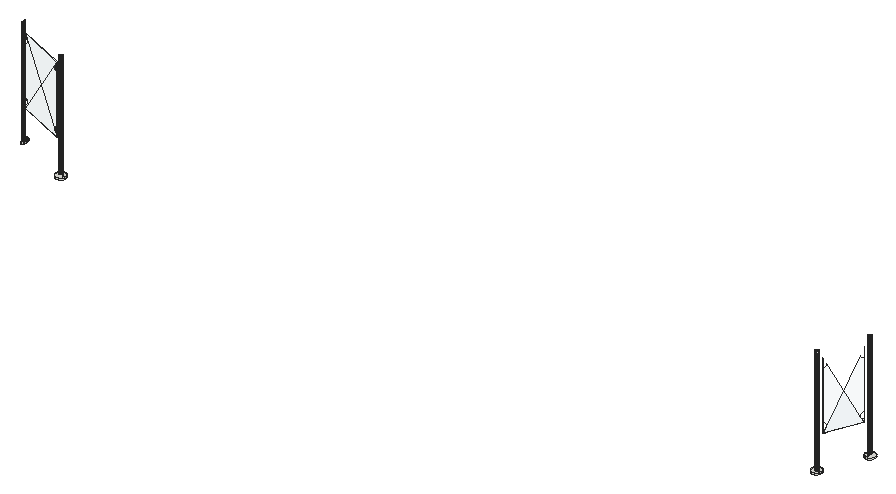
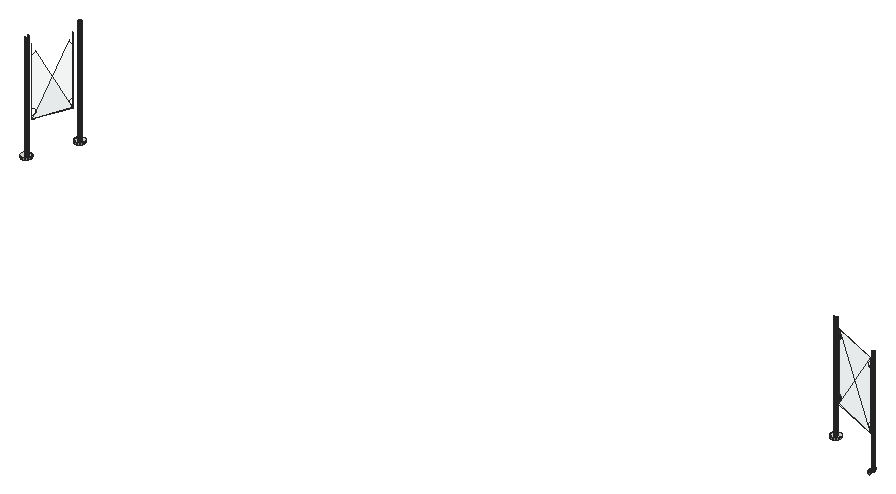
# SketchUp Ruby script. Lengths in inches.
U = 1.inch
M = Sketchup.active_model
def pt(a) = Geom::Point3d.new(a.map { |v| v * U })
def face(e, loops, mat)
  f = e.add_face(loops[0].map { |a| pt(a) })
  loops[1..].each { |l| e.add_face(l.map { |a| pt(a) }).erase! }
  f.material = f.back_material = mat if mat
  f
end
# faces: each face lists its corners as indices into pts; further lists are holes
def faces(e, pts, list, mat = nil) = list.each { |f| face(e, (f[0].is_a?(Array) ? f : [f]).map { |l| l.map { |i| pts[i] } }, mat) }
# xy, xz, yz: faces in a plane at the given z, y or x. An outline is a flat list of corners, or four numbers for a rectangle; further outlines are holes
def ring(l) = l.size == 4 ? [[l[0], l[1]], [l[2], l[1]], [l[2], l[3]], [l[0], l[3]]] : l.each_slice(2).to_a
def flat(e, list, mat, &to3) = list.each { |f| face(e, (f[0].is_a?(Array) ? f : [f]).map { |l| ring(l).map { |u, v| to3.(u, v) } }, mat) }
def xy(e, z, list, mat = nil) = flat(e, list, mat) { |x, y| [x, y, z] }
def xz(e, y, list, mat = nil) = flat(e, list, mat) { |x, z| [x, y, z] }
def yz(e, x, list, mat = nil) = flat(e, list, mat) { |y, z| [x, y, z] }
def lines(e, pts, list) = list.each { |a, b| e.add_line(pt(pts[a]), pt(pts[b])) }
# prism: a flat outline (further loops are holes) pulled along v
def prism(e, loops, v, mat = nil)
  f = face(e, loops, mat); d = Geom::Vector3d.new(v.map { |x| x * U })
  f.pushpull(f.normal.samedirection?(d) ? d.length : -d.length)
end
def box(e, o, s, mat = nil) = prism(e, [[o, [o[0] + s[0], o[1], o[2]], [o[0] + s[0], o[1] + s[1], o[2]], [o[0], o[1] + s[1], o[2]]]], [0, 0, s[2]], mat)
def at(x, y, z, deg = 0) = Geom::Transformation.translation(pt([x, y, z])) * Geom::Transformation.rotation(ORIGIN, Z_AXIS, deg.degrees)
def axes(o, x, y, z) = Geom::Transformation.new([*x, 0, *y, 0, *z, 0, *pt(o).to_a, 1])
def part(name) = M.definitions.add(name)
# library, detail: a bought-in or finely detailed component or shape, given as its bounding box
def library(name, o, s) = part(name).tap { |d| box(d.entities, o, s) }
def detail(e, o, s) = box(e.add_group.entities, o, s)
def put(e, d, t, mat = nil) = e.add_instance(d, t).tap { |i| i.material = mat if mat }
def group(e, t, mat = nil) = e.add_group.tap { |g| g.transformation = t; g.material = mat if mat }.entities
root = M.entities
M.materials.add("Glass_Safety_01").color = [204, 235, 244]
M.materials["Glass_Safety_01"].alpha = 0.1
M.materials.add("[Color_000]").color = [255, 255, 255]
xy(root,321.27,[[[632.17,624.43,632.57,624.51,632.94,624.69,633.25,624.97,633.47,625.31,633.6,625.7,633.63,626.11,633.55,626.51,633.36,626.88,633.09,627.1875,632.74,627.41,632.35,627.54,631.94,627.57,631.54,627.49,631.17,627.3,630.87,627.03,630.64,626.6875,630.62,626.625,630.51,626.3,630.49,625.89,630.57,625.48,630.75,625.11,631.03,624.81,631.37,624.58,631.76,624.45],[632.1,625.37,631.9375,625.38,631.78,625.43,631.64,625.52,631.54,625.64,631.46,625.79,631.43,625.95,631.4375,626.12,631.48,626.25,631.49,626.27,631.58,626.41,631.7,626.52,631.85,626.59,632.01,626.625,632.18,626.62,632.33,626.5625,632.47,626.47,632.58,626.35,632.65,626.2,632.69,626.04,632.68,625.88,632.63,625.75,632.625,625.72,632.53,625.59,632.41,625.48,632.26,625.4]],[[883.4375,625.03,883.84,625.11,884.21,625.3,884.51,625.57,884.74,625.91,884.87,626.3,884.9,626.71,884.8125,627.12,884.63,627.48,884.36,627.79,884.01,628.02,883.62,628.15,883.4,628.16,883.21,628.17,882.81,628.09,882.44,627.91,882.13,627.63,881.91,627.29,881.78,626.9,881.75,626.49,881.84,626.09,882.02,625.72,882.23,625.48,882.29,625.41,882.64,625.18,883.03,625.05],[883.37,625.97,883.21,625.98,883.05,626.03,882.91,626.125,882.8,626.25,882.73,626.39,882.7,626.54,882.7,626.56,882.71,626.72,882.76,626.875,882.85,627.01,882.9375,627.09,882.97,627.12,883.12,627.2,883.28,627.23,883.44,627.22,883.6,627.17,883.74,627.08,883.85,626.95,883.92,626.81,883.95,626.65,883.94,626.48,883.89,626.33,883.8,626.1875,883.68,626.08,883.53,626.01]],[633.49,625.37,633.6,625.7,633.63,626.11,633.55,626.51,633.36,626.88,633.09,627.1875,632.74,627.41,632.35,627.54,631.94,627.57,631.54,627.49,631.17,627.3,630.87,627.03,630.64,626.6875,630.62,626.625,631.48,626.25,631.49,626.27,631.58,626.41,631.7,626.52,631.85,626.59,632.01,626.625,632.18,626.62,632.33,626.5625,632.47,626.47,632.58,626.35,632.65,626.2,632.69,626.04,632.68,625.88,632.63,625.75],[882.23,625.48,882.7,626.54,882.7,626.56,882.71,626.72,882.76,626.875,882.85,627.01,882.9375,627.09,883.4,628.16,883.21,628.17,882.81,628.09,882.44,627.91,882.13,627.63,881.91,627.29,881.78,626.9,881.75,626.49,881.84,626.09,882.02,625.72],[632.63,625.75,632.68,625.88,632.69,626.04,632.65,626.2,632.58,626.35,632.47,626.47,632.33,626.5625,632.18,626.62,632.01,626.625,631.85,626.59,631.7,626.52,631.58,626.41,631.49,626.27,631.48,626.25],
  [882.7,626.54,882.9375,627.09,882.85,627.01,882.76,626.875,882.71,626.72,882.7,626.56],[[889.33,639.9375,889.73,640.02,890.1,640.2,890.41,640.48,890.63,640.82,890.76,641.21,890.79,641.62,890.7,642.02,890.52,642.39,890.25,642.7,889.9,642.92,889.51,643.05,889.1,643.08,888.7,643,888.33,642.8125,888.03,642.54,887.8,642.2,887.67,641.81,887.64,641.4,887.73,640.99,887.91,640.625,888.18,640.32,888.53,640.09,888.92,639.96],[889.26,640.88,889.1,640.89,888.97,640.93,888.94,640.94,888.8,641.03,888.69,641.15,888.62,641.3,888.59,641.46,888.6,641.625,888.65,641.78,888.74,641.92,888.86,642.03,889.01,642.1,889.17,642.14,889.33,642.125,889.47,642.08,889.49,642.07,889.63,641.98,889.74,641.86,889.8125,641.71,889.84,641.55,889.83,641.39,889.78,641.23,889.69,641.1,889.57,640.99,889.42,640.91]],[888.59,640.07,888.97,640.93,888.94,640.94,888.8,641.03,888.69,641.15,888.62,641.3,888.59,641.46,888.6,641.625,888.65,641.78,888.74,641.92,888.86,642.03,889.01,642.1,889.17,642.14,889.33,642.125,889.47,642.08,889.84,642.94,889.51,643.05,889.1,643.08,888.7,643,888.33,642.8125,888.03,642.54,887.8,642.2,887.67,641.81,887.64,641.4,887.73,640.99,887.91,640.625,888.18,640.32,888.53,640.09],[888.97,640.93,889.47,642.08,889.33,642.125,889.17,642.14,889.01,642.1,888.86,642.03,888.74,641.92,888.65,641.78,888.6,641.625,888.59,641.46,888.62,641.3,888.69,641.15,888.8,641.03,888.94,640.94]])
xy(root,321.27,[[883.37,625.97,883.53,626.01,883.68,626.08,883.8,626.1875,883.89,626.33,883.94,626.48,883.95,626.65,883.92,626.81,883.85,626.95,883.74,627.08,883.6,627.17,883.44,627.22,883.28,627.23,883.12,627.2,882.97,627.12,882.9375,627.09,882.85,627.01,882.76,626.875,882.71,626.72,882.7,626.56,882.7,626.54,882.73,626.39,882.8,626.25,882.91,626.125,883.05,626.03,883.21,625.98]],"[Color_000]")
xy(root,321.86,[[632.17,624.43,632.57,624.51,632.94,624.69,633.25,624.97,633.47,625.31,633.6,625.7,633.63,626.11,633.55,626.51,633.36,626.88,633.09,627.1875,632.74,627.41,632.35,627.54,631.94,627.57,631.54,627.49,631.17,627.3,630.87,627.03,630.64,626.6875,630.51,626.3,630.49,625.89,630.57,625.48,630.75,625.11,631.03,624.81,631.37,624.58,631.76,624.45],[883.4375,625.03,883.84,625.11,884.21,625.3,884.51,625.57,884.74,625.91,884.87,626.3,884.9,626.71,884.8125,627.12,884.63,627.48,884.36,627.79,884.01,628.02,883.62,628.15,883.21,628.17,882.81,628.09,882.44,627.91,882.13,627.63,881.91,627.29,881.78,626.9,881.75,626.49,881.84,626.09,882.02,625.72,882.29,625.41,882.64,625.18,883.03,625.05],[889.33,639.9375,889.73,640.02,890.1,640.2,890.41,640.48,890.63,640.82,890.76,641.21,890.79,641.62,890.7,642.02,890.52,642.39,890.25,642.7,889.9,642.92,889.51,643.05,889.1,643.08,888.7,643,888.33,642.8125,888.03,642.54,887.8,642.2,887.67,641.81,887.64,641.4,887.73,640.99,887.91,640.625,888.18,640.32,888.53,640.09,888.92,639.96]])
xy(root,331.9,[[630.38,626.62,614.1875,633.67,614.27,633.85],[630.38,626.62,614.27,633.85,630.46,626.8],[884.14,628.4,883.96,628.47,888.67,639.87],[883.96,628.47,888.49,639.9375,888.67,639.87]],"Glass_Safety_01")
p = [[633.6,625.7,321.27],[633.63,626.11,321.27],[633.63,626.11,321.86],[633.6,625.7,321.86],[630.51,626.3,321.27],[630.49,625.89,321.27],
  [630.49,625.89,321.86],[630.51,626.3,321.86],[632.68,625.88,321.27],[632.69,626.04,321.27],[632.69,626.04,357.27],[632.68,625.88,357.27],
  [884.74,625.91,321.27],[884.87,626.3,321.27],[884.87,626.3,321.86],[884.74,625.91,321.86],[631.4375,626.12,321.27],[631.43,625.95,321.27],
  [631.43,625.95,357.27],[631.4375,626.12,357.27],[632.65,626.2,321.27],[632.65,626.2,357.27],[882.91,626.125,321.27],[883.05,626.03,321.27],
  [883.05,626.03,357.27],[882.91,626.125,357.27],[883.21,625.98,321.27],[883.21,625.98,357.27],[883.37,625.97,321.27],[883.37,625.97,357.27],
  [883.53,626.01,321.27],[883.53,626.01,357.27],[883.68,626.08,321.27],[883.68,626.08,357.27],[631.49,626.27,321.27],[631.48,626.25,321.27],
  [631.49,626.27,357.27],[633.55,626.51,321.27],[633.55,626.51,321.86],[881.75,626.49,321.27],[881.84,626.09,321.27],[881.84,626.09,321.86],
  [881.75,626.49,321.86],[882.8,626.25,321.27],[882.8,626.25,357.27],[883.8,626.1875,321.27],[883.8,626.1875,357.27],[632.58,626.35,321.27],
  [632.58,626.35,357.27],[882.73,626.39,321.27],[882.73,626.39,357.27],[883.89,626.33,321.27],[883.89,626.33,357.27],[630.64,626.6875,321.27],
  [630.62,626.625,321.27],[630.64,626.6875,321.86],[631.58,626.41,321.27],[631.58,626.41,357.27],[883.94,626.48,321.27],[883.94,626.48,357.27],
  [884.9,626.71,321.27],[884.9,626.71,321.86],[631.7,626.52,321.27],[631.7,626.52,357.27],[632.47,626.47,321.27],[632.47,626.47,357.27],
  [882.7,626.56,321.27],[882.7,626.54,321.27],[882.7,626.56,357.27],[631.85,626.59,321.27],[631.85,626.59,357.27],[632.33,626.5625,321.27],
  [632.33,626.5625,357.27],[633.36,626.88,321.27],[633.36,626.88,321.86],[881.78,626.9,321.27],[881.78,626.9,321.86],[883.95,626.65,321.27],
  [883.95,626.65,357.27],[632.01,626.625,321.27],[632.01,626.625,357.27],[632.18,626.62,321.27],[632.18,626.62,357.27],[882.71,626.72,321.27],
  [882.71,626.72,357.27],[883.92,626.81,321.27],[883.92,626.81,357.27],[630.87,627.03,321.27],[630.87,627.03,321.86],[882.76,626.875,321.27],
  [882.76,626.875,357.27],[884.8125,627.12,321.27],[884.8125,627.12,321.86],[883.85,626.95,321.27],[883.85,626.95,357.27],[633.09,627.1875,321.27],
  [633.09,627.1875,321.86],[881.91,627.29,321.27],[881.91,627.29,321.86],[882.85,627.01,321.27],[882.85,627.01,357.27],[631.17,627.3,321.27],
  [631.17,627.3,321.86],[882.97,627.12,321.27],[882.9375,627.09,321.27],[882.97,627.12,357.27],[883.74,627.08,321.27],[883.74,627.08,357.27],
  [883.12,627.2,321.27],[883.12,627.2,357.27],[883.6,627.17,321.27],[883.6,627.17,357.27],[884.63,627.48,321.27],[884.63,627.48,321.86],
  [632.74,627.41,321.27],[632.74,627.41,321.86],[883.28,627.23,321.27],[883.28,627.23,357.27],[883.44,627.22,321.27],[883.44,627.22,357.27],
  [631.54,627.49,321.27],[631.54,627.49,321.86],[882.13,627.63,321.27],[882.13,627.63,321.86],[632.35,627.54,321.27],[632.35,627.54,321.86],
  [631.94,627.57,321.27],[631.94,627.57,321.86],[884.36,627.79,321.27],[884.36,627.79,321.86],[882.44,627.91,321.27],[882.44,627.91,321.86],
  [884.01,628.02,321.27],[884.01,628.02,321.86],[882.81,628.09,321.27],[882.81,628.09,321.86],[883.62,628.15,321.27],[883.62,628.15,321.86],
  [883.21,628.17,321.27],[883.21,628.17,321.86],[883.4,628.16,321.27],[612.9375,633.0625,321.27],[613.3,633.25,321.27],[613.3,633.25,321.86],
  [612.9375,633.0625,321.86],[613.61,633.52,321.27],[613.61,633.52,321.86],[613.84,633.86,321.27],[613.84,633.86,321.86],[613.86,633.92,321.27],
  [613.97,634.25,321.27],[613.97,634.25,321.86],[612.77,634.03,321.27],[612.9,634.14,321.27],[612.9,634.14,357.27],[612.77,634.03,357.27],
  [612.99,634.27,321.27],[612.99,634.27,357.27],[613,634.3,321.27],[613.04,634.43,321.27],[613.04,634.43,357.27],[613.99,634.66,321.27],
  [613.99,634.66,321.86],[613.05,634.59,321.27],[613.05,634.59,357.27],[613.02,634.76,321.27],[613.02,634.76,357.27],[613.91,635.06,321.27],
  [613.91,635.06,321.86],[612.94,634.9,321.27],[612.94,634.9,357.27],[612.83,635.03,321.27],[612.83,635.03,357.27],[613.73,635.43,321.27],
  [613.73,635.43,321.86],[613.45,635.74,321.27],[613.45,635.74,321.86],[613.11,635.97,321.27],[613.11,635.97,321.86],[612.72,636.1,321.27],
  [612.72,636.1,321.86],[888.92,639.96,321.27],[889.33,639.9375,321.27],[889.33,639.9375,321.86],[888.92,639.96,321.86],[888.53,640.09,321.27],
  [888.59,640.07,321.27],[888.53,640.09,321.86],[888.18,640.32,321.27],[888.18,640.32,321.86],[887.91,640.625,321.27],[887.91,640.625,321.86],
  [887.73,640.99,321.27],[887.73,640.99,321.86],[888.8,641.03,321.27],[888.94,640.94,321.27],[888.94,640.94,357.27],[888.8,641.03,357.27],
  [888.97,640.93,321.27],[889.1,640.89,321.27],[889.1,640.89,357.27],[889.26,640.88,321.27],[889.26,640.88,357.27],[887.64,641.4,321.27],
  [887.64,641.4,321.86],[888.69,641.15,321.27],[888.69,641.15,357.27],[888.62,641.3,321.27],[888.62,641.3,357.27],[888.59,641.46,321.27],
  [888.59,641.46,357.27],[887.67,641.81,321.27],[887.67,641.81,321.86],[888.6,641.625,321.27],[888.6,641.625,357.27],[888.65,641.78,321.27],
  [888.65,641.78,357.27],[887.8,642.2,321.27],[887.8,642.2,321.86],[888.74,641.92,321.27],[888.74,641.92,357.27],[888.86,642.03,321.27],
  [888.86,642.03,357.27],[889.01,642.1,321.27],[889.01,642.1,357.27],[889.17,642.14,321.27],[889.17,642.14,357.27],[888.03,642.54,321.27],
  [888.03,642.54,321.86],[888.33,642.8125,321.27],[888.33,642.8125,321.86],[888.7,643,321.27],[888.7,643,321.86],[889.1,643.08,321.27],
  [889.1,643.08,321.86],[614.1875,633.67,351.28],[614.1875,633.67,335.125],[614.4375,633.5625,335.09],[614.67,633.46,334.98],[614.875,633.375,334.8125],
  [615.03,633.31,334.59],[615.13,633.26,334.34],[615.16,633.25,334.0625],[615.13,633.26,333.79],[615.03,633.31,333.53],[614.875,633.375,333.3125],
  [614.67,633.46,333.14],[614.4375,633.5625,333.04],[614.1875,633.67,333],[614.1875,633.67,331.9],[630.38,626.62,354.51],[614.1875,633.67,354.51],
  [614.1875,633.67,353.41],[614.4375,633.5625,353.37],[614.67,633.46,353.27],[614.875,633.375,353.1],[615.03,633.31,352.88],[615.13,633.26,352.62],
  [615.16,633.25,352.35],[615.13,633.26,352.07],[615.03,633.31,351.81],[614.875,633.375,351.59],[614.67,633.46,351.43],[614.4375,633.5625,351.32],
  [630.38,626.62,331.9],[630.38,626.62,333],[630.21,626.69,333],[629.96,626.8,333.04],[629.73,626.91,333.14],[629.52,626.99,333.3125],
  [629.37,627.0625,333.53],[629.27,627.1,333.79],[629.24,627.12,334.0625],[629.27,627.1,334.34],[629.37,627.0625,334.59],[629.52,626.99,334.8125],
  [629.73,626.91,334.98],[629.96,626.8,335.09],[630.21,626.69,335.125],[630.38,626.62,335.125],[630.38,626.62,351.28],[630.21,626.69,351.28],
  [629.96,626.8,351.32],[629.73,626.91,351.43],[629.52,626.99,351.59],[629.37,627.0625,351.81],[629.27,627.1,352.07],[629.24,627.12,352.35],
  [629.27,627.1,352.62],[629.37,627.0625,352.88],[629.52,626.99,353.1],[629.73,626.91,353.27],[629.96,626.8,353.37],[630.21,626.69,353.41],
  [630.38,626.62,353.41],[630.46,626.8,331.9],[630.46,626.8,333],[630.46,626.8,335.125],[630.46,626.8,351.28],[630.46,626.8,353.41],
  [630.46,626.8,354.51],[614.27,633.85,331.9],[614.27,633.85,333],[614.52,633.74,333.04],[614.75,633.64,333.14],[614.95,633.55,333.3125],
  [615.11,633.49,333.53],[615.21,633.44,333.79],[615.24,633.43,334.0625],[615.21,633.44,334.34],[615.11,633.49,334.59],[614.95,633.55,334.8125],
  [614.75,633.64,334.98],[614.52,633.74,335.09],[614.27,633.85,335.125],[614.27,633.85,351.28],[614.52,633.74,351.32],[614.75,633.64,351.43],
  [614.95,633.55,351.59],[615.11,633.49,351.81],[615.21,633.44,352.07],[615.24,633.43,352.35],[615.21,633.44,352.62],[615.11,633.49,352.88],
  [614.95,633.55,353.1],[614.75,633.64,353.27],[614.52,633.74,353.37],[614.27,633.85,353.41],[614.27,633.85,354.51],[630.29,626.875,335.125],
  [630.04,626.98,335.09],[629.8,627.09,334.98],[629.6,627.17,334.8125],[629.45,627.24,334.59],[629.35,627.28,334.34],[629.32,627.3,334.0625],
  [629.35,627.28,333.79],[629.45,627.24,333.53],[629.6,627.17,333.3125],[629.8,627.09,333.14],[630.04,626.98,333.04],[630.29,626.875,333],
  [630.29,626.875,353.41],[630.04,626.98,353.37],[629.8,627.09,353.27],[629.6,627.17,353.1],[629.45,627.24,352.88],[629.35,627.28,352.62],
  [629.32,627.3,352.35],[629.35,627.28,352.07],[629.45,627.24,351.81],[629.6,627.17,351.59],[629.8,627.09,351.43],[630.04,626.98,351.32],
  [630.29,626.875,351.28],[883.96,628.47,331.9],[884.14,628.4,331.9],[884.14,628.4,333],[884.14,628.4,335.125],[884.14,628.4,351.28],
  [884.14,628.4,353.41],[884.14,628.4,354.51],[883.96,628.47,354.51],[883.96,628.47,353.41],[883.96,628.47,351.28],[883.96,628.47,335.125],
  [883.96,628.47,333],[884.44,629.16,333.4],[884.42,629.09,333.3125],[884.33,628.89,333.14],[884.24,628.65,333.04],[888.2,638.67,352.16],
  [884.51,629.34,333.76],[884.48,629.25,333.53],[888.67,639.87,331.9],[888.67,639.87,333],[888.58,639.64,333],[888.48,639.38,333.04],
  [888.39,639.15,333.14],[888.31,638.94,333.3125],[888.25,638.78,333.53],[888.21,638.6875,333.79],[888.19,638.65,334.0625],[888.21,638.6875,334.34],
  [888.25,638.78,334.59],[888.31,638.94,334.8125],[888.39,639.15,334.98],[888.48,639.38,335.09],[888.58,639.64,335.125],[888.67,639.87,335.125],
  [888.67,639.87,351.28],[888.58,639.64,351.28],[888.48,639.38,351.32],[888.39,639.15,351.43],[888.31,638.94,351.59],[888.25,638.78,351.8125],
  [888.21,638.6875,352.07],[884.06,628.72,351.32],[884.15,628.96,351.43],[884.23,629.17,351.59],[884.29,629.32,351.8125],[884.33,629.42,352.07],
  [884.35,629.46,352.35],[884.33,629.42,352.62],[884.33,629.41,352.65],[888.02,638.75,334.25],[888.01,638.72,334.0625],[888.02,638.76,333.79],
  [888.0625,638.86,333.53],[888.125,639.01,333.3125],[888.21,639.22,333.14],[888.25,639.33,333.09],[888.49,639.9375,331.9],[884.06,628.72,333.04],
  [884.15,628.96,333.14],[884.23,629.17,333.3125],[884.29,629.32,333.53],[884.33,629.42,333.79],[884.35,629.46,334.0625],[884.33,629.42,334.34],
  [884.29,629.32,334.59],[884.23,629.17,334.8125],[884.15,628.96,334.98],[884.06,628.72,335.09],[888.3,639.46,333.04],[888.4,639.71,333],
  [888.49,639.9375,333],[888.49,639.9375,335.125],[888.49,639.9375,351.28],[888.49,639.9375,353.41],[888.49,639.9375,354.51],[888.67,639.87,354.51],
  [888.67,639.87,353.41]]
faces(root,p,[[0,1,2,3],[4,5,6,7],[12,13,14,15],[1,37,38,2],[39,40,41,42],[53,54,4,7,55],[13,60,61,14],[37,73,74,38],
  [75,39,42,76],[87,53,55,88],[60,91,92,61],[73,95,96,74],[97,75,76,98],[101,87,88,102],[91,112,113,92],[95,114,115,96],
  [120,101,102,121],[122,97,98,123],[114,124,125,115],[126,120,121,127],[124,126,127,125],[112,128,129,113],[130,122,123,131],[128,132,133,129],
  [134,130,131,135],[132,136,137,133],[138,134,135,139],[136,140,138,139,137],[141,142,143,144],[142,145,146,143],[145,147,148,146],[147,149,150,151,148],
  [150,161,162,151],[161,167,168,162],[167,173,174,168],[173,175,176,174],[175,177,178,176],[177,179,180,178],[181,182,183,184],[185,186,181,184,187],
  [188,185,187,189],[190,188,189,191],[192,190,191,193],[203,192,193,204],[211,203,204,212],[217,211,212,218],[227,217,218,228],[229,227,228,230],
  [231,229,230,232],[233,231,232,234]])
faces(root,p,[[8,9,10,11],[16,17,18,19],[9,20,21,10],[22,23,24,25],[23,26,27,24],[26,28,29,27],[28,30,31,29],[30,32,33,31],
  [34,35,16,19,36],[43,22,25,44],[32,45,46,33],[20,47,48,21],[49,43,44,50],[45,51,52,46],[56,34,36,57],[51,58,59,52],
  [62,56,57,63],[47,64,65,48],[66,67,49,50,68],[69,62,63,70],[64,71,72,65],[58,77,78,59],[79,69,70,80],[81,79,80,82],
  [71,81,82,72],[83,66,68,84],[77,85,86,78],[89,83,84,90],[85,93,94,86],[99,89,90,100],[103,104,99,100,105],[93,106,107,94],
  [108,103,105,109],[106,110,111,107],[116,108,109,117],[118,116,117,119],[110,118,119,111],[152,153,154,155],[153,156,157,154],[156,158,159,160,157],
  [159,163,164,160],[163,165,166,164],[165,169,170,166],[169,171,172,170],[194,195,196,197],[195,198,199,200,196],[199,201,202,200],[205,194,197,206],
  [207,205,206,208],[209,207,208,210],[213,209,210,214],[215,213,214,216],[219,215,216,220],[221,219,220,222],[223,221,222,224],[225,223,224,226]],"[Color_000]")
faces(root,p,[[235,236,237,238,239,240,241,242,243,244,245,246,247,248,249,250,251,252,253,254,255,256,257,258,259,260,261,262,263],[264,265,266,267,268,269,270,271,272,273,274,275,276,277,278,279,280,281,282,283,284,285,286,287,288,289,290,291,292,293,294,250,249],[264,295,296,297,298,299,300,250,294,280,279,265],[301,302,303,304,305,306,307,308,309,310,311,312,313,314,315,316,317,318,319,320,321,322,323,324,325,326,327,328,295],[298,297,329,330,331,332,333,334,335,336,337,338,339,340,341,296,295,328,300,299,342,343,344,345,346,347,348,349,350,351,352,353,354],[355,356,357,358,359,360,361,362,363,364,365,366],[356,367,368,369,370,357],[371,372,373,367,356,374,375,376,377,378,379,380,381,382,383,384,385,386,387,388,389,390,391,392,393,394,395,396],
  [365,364,397,398,399,400,401,402,403,404,405,406,407,408,409,410,411,412,355,366,413,414,415,416,417,418,419,420,421,422,423],[301,249,248,236,235,252,251,328,327,315,314,302],[412,411,424,425,426],[374,412,426,427,428,429,430,431,432,390,389,375]],"Glass_Safety_01")
